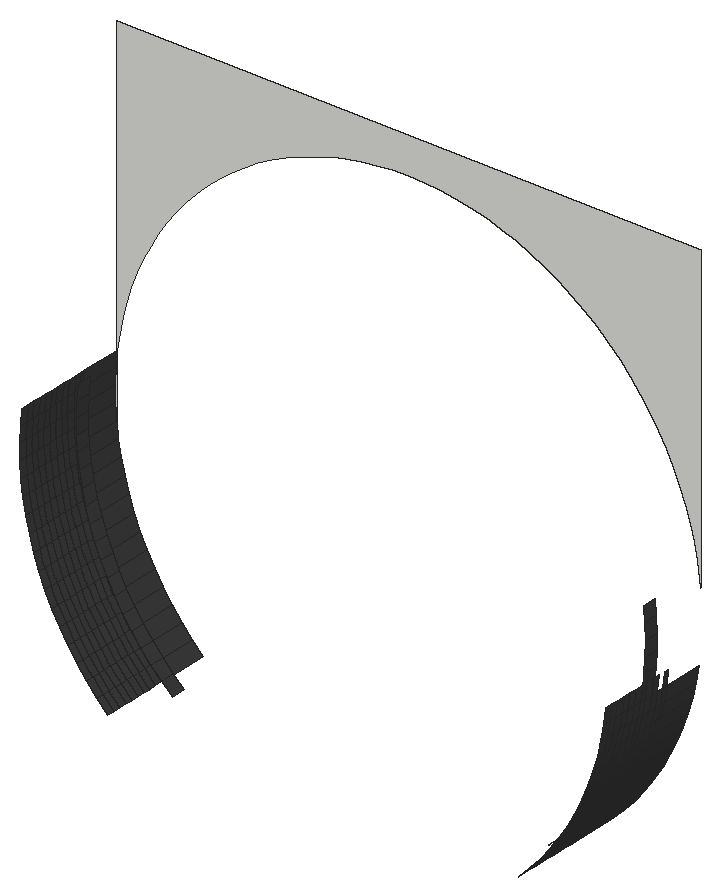
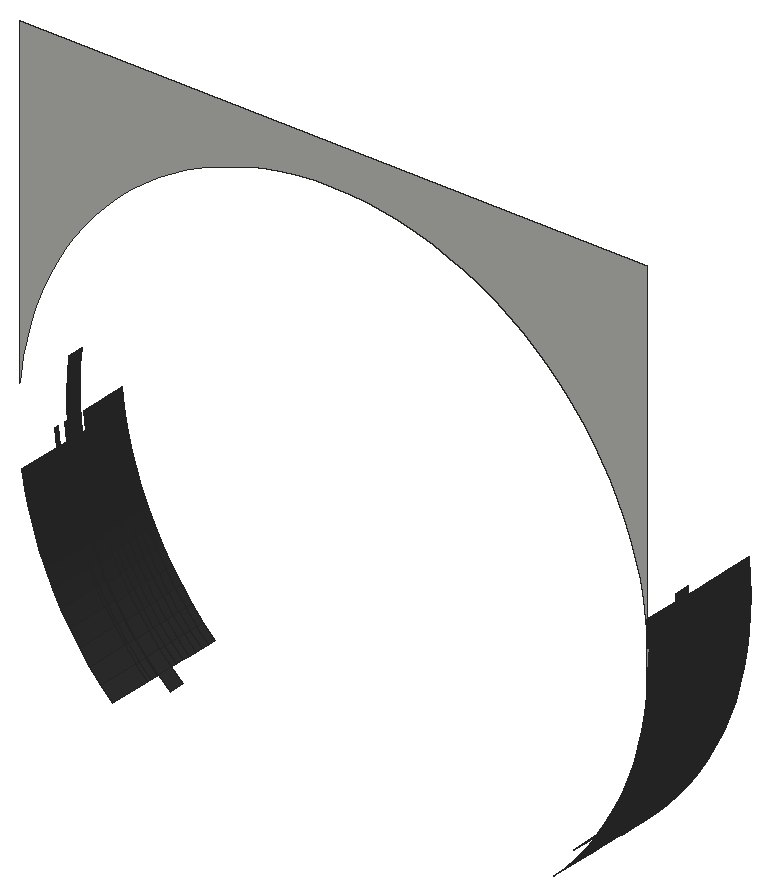
# SketchUp Ruby script. Lengths in inches.
U = 1.inch
M = Sketchup.active_model
def pt(a) = Geom::Point3d.new(a.map { |v| v * U })
def face(e, loops, mat)
  f = e.add_face(loops[0].map { |a| pt(a) })
  loops[1..].each { |l| e.add_face(l.map { |a| pt(a) }).erase! }
  f.material = f.back_material = mat if mat
  f
end
# faces: each face lists its corners as indices into pts; further lists are holes
def faces(e, pts, list, mat = nil) = list.each { |f| face(e, (f[0].is_a?(Array) ? f : [f]).map { |l| l.map { |i| pts[i] } }, mat) }
# xy, xz, yz: faces in a plane at the given z, y or x. An outline is a flat list of corners, or four numbers for a rectangle; further outlines are holes
def ring(l) = l.size == 4 ? [[l[0], l[1]], [l[2], l[1]], [l[2], l[3]], [l[0], l[3]]] : l.each_slice(2).to_a
def flat(e, list, mat, &to3) = list.each { |f| face(e, (f[0].is_a?(Array) ? f : [f]).map { |l| ring(l).map { |u, v| to3.(u, v) } }, mat) }
def xy(e, z, list, mat = nil) = flat(e, list, mat) { |x, y| [x, y, z] }
def xz(e, y, list, mat = nil) = flat(e, list, mat) { |x, z| [x, y, z] }
def yz(e, x, list, mat = nil) = flat(e, list, mat) { |y, z| [x, y, z] }
def lines(e, pts, list) = list.each { |a, b| e.add_line(pt(pts[a]), pt(pts[b])) }
# prism: a flat outline (further loops are holes) pulled along v
def prism(e, loops, v, mat = nil)
  f = face(e, loops, mat); d = Geom::Vector3d.new(v.map { |x| x * U })
  f.pushpull(f.normal.samedirection?(d) ? d.length : -d.length)
end
def box(e, o, s, mat = nil) = prism(e, [[o, [o[0] + s[0], o[1], o[2]], [o[0] + s[0], o[1] + s[1], o[2]], [o[0], o[1] + s[1], o[2]]]], [0, 0, s[2]], mat)
def at(x, y, z, deg = 0) = Geom::Transformation.translation(pt([x, y, z])) * Geom::Transformation.rotation(ORIGIN, Z_AXIS, deg.degrees)
def axes(o, x, y, z) = Geom::Transformation.new([*x, 0, *y, 0, *z, 0, *pt(o).to_a, 1])
def part(name) = M.definitions.add(name)
# library, detail: a bought-in or finely detailed component or shape, given as its bounding box
def library(name, o, s) = part(name).tap { |d| box(d.entities, o, s) }
def detail(e, o, s) = box(e.add_group.entities, o, s)
def put(e, d, t, mat = nil) = e.add_instance(d, t).tap { |i| i.material = mat if mat }
def group(e, t, mat = nil) = e.add_group.tap { |g| g.transformation = t; g.material = mat if mat }.entities
root = M.entities
M.materials.add("[Color M07]").color = [58, 58, 58]
xz(root,24,[[27.46,301.2,27.46,312.54,27.31,310.86,27.18,307.68,27.23,304.49,27.45,301.3125],[27.46,312.54,27.46,373.6875,145.46,373.6875,145.46,312.54,145.32,314.03,144.86,317.1875,144.22,320.31,143.42,323.39,142.46,326.43,141.33,329.41,140.05,332.33,138.61,335.17,137.02,337.93,135.28,340.6,133.4,343.17,131.39,345.64,129.25,348,126.98,350.24,124.6,352.36,122.1,354.34,119.51,356.1875,116.81,357.89,114.04,359.45,111.18,360.85,108.24,362.1,105.25,363.19,102.2,364.12,99.11,364.88,95.98,365.48,92.82,365.91,89.65,366.16,86.46,366.25,83.28,366.16,80.1,365.91,76.94,365.48,73.8125,364.88,70.72,364.12,67.67,363.19,64.68,362.1,61.75,360.85,58.89,359.45,56.11,357.89,53.42,356.1875,50.82,354.34,48.32,352.36,45.94,350.24,43.67,348,41.53,345.64,39.52,343.17,37.64,340.6,35.9,337.93,34.3125,335.17,32.875,332.33,31.59,329.41,30.46,326.43,29.5,323.39,28.7,320.31,28.06,317.1875,27.6,314.03]])
p = [[48.46,14.875,263.875],[46.2,14.875,265.98],[46.2,12,265.98],[48.46,12,263.875],[126.72,14.875,265.98],[124.46,14.875,263.875],
  [124.46,12,263.875],[126.72,12,265.98],[44.92,0,264.68],[44.92,1.5,264.68],[42.7,1.5,266.97],[42.7,0,266.97],
  [130.22,0,266.97],[130.22,1.5,266.97],[128.01,1.5,264.68],[128.01,0,264.68],[44.92,3,264.68],[42.7,3,266.97],
  [130.22,3,266.97],[128.01,3,264.68],[44.92,4.5,264.68],[42.7,4.5,266.97],[130.22,4.5,266.97],[128.01,4.5,264.68],
  [44.92,6,264.68],[42.7,6,266.97],[130.22,6,266.97],[128.01,6,264.68],[44.92,7.5,264.68],[42.7,7.5,266.97],
  [130.22,7.5,266.97],[128.01,7.5,264.68],[44.92,9,264.68],[42.7,9,266.97],[130.22,9,266.97],[128.01,9,264.68],
  [44.92,10.5,264.68],[42.7,10.5,266.97],[130.22,10.5,266.97],[128.01,10.5,264.68],[44.92,12,264.68],[42.7,12,266.97],
  [130.22,12,266.97],[128.01,12,264.68],[44.92,13.5,264.68],[42.7,13.5,266.97],[130.22,13.5,266.97],[128.01,13.5,264.68],
  [44.92,15,264.68],[42.7,15,266.97],[130.22,15,266.97],[128.01,15,264.68],[44.92,15.8125,264.68],[42.7,15.8125,266.97],
  [130.22,15.8125,266.97],[128.01,15.8125,264.68],[42.7,24,266.97],[44.92,24,264.68],[128.01,24,264.68],[130.22,24,266.97],
  [44.05,14.875,268.2],[44.05,12,268.2],[128.87,14.875,268.2],[128.87,12,268.2],[40.62,1.5,269.375],[40.62,0,269.375],
  [132.31,0,269.375],[132.31,1.5,269.375],[40.62,3,269.375],[132.31,3,269.375],[40.62,4.5,269.375],[132.31,4.5,269.375],
  [40.62,6,269.375],[132.31,6,269.375],[40.62,7.5,269.375],[132.31,7.5,269.375],[40.62,9,269.375],[132.31,9,269.375],
  [40.62,10.5,269.375],[132.31,10.5,269.375],[40.62,12,269.375],[132.31,12,269.375],[40.62,13.5,269.375],[132.31,13.5,269.375],
  [40.62,15,269.375],[132.31,15,269.375],[40.62,15.8125,269.375],[132.31,15.8125,269.375],[40.62,24,269.375],[132.31,24,269.375],
  [42.03,14.875,270.54],[42.03,12,270.54],[130.89,14.875,270.54],[130.89,12,270.54],[38.66,1.5,271.89],[38.66,0,271.89],
  [134.26,0,271.89],[134.26,1.5,271.89],[38.66,3,271.89],[134.26,3,271.89],[38.66,4.5,271.89],[134.26,4.5,271.89],
  [38.66,6,271.89],[134.26,6,271.89],[38.66,7.5,271.89],[134.26,7.5,271.89],[38.66,9,271.89],[134.26,9,271.89],
  [38.66,10.5,271.89],[134.26,10.5,271.89],[38.66,12,271.89],[134.26,12,271.89],[38.66,13.5,271.89],[134.26,13.5,271.89],
  [38.66,15,271.89],[134.26,15,271.89],[38.66,15.8125,271.89],[134.26,15.8125,271.89],[38.66,24,271.89],[134.26,24,271.89],
  [40.14,14.875,272.98],[40.14,12,272.98],[132.78,14.875,272.98],[132.78,12,272.98],[36.85,1.5,274.51],[36.85,0,274.51],
  [136.07,0,274.51],[136.07,1.5,274.51],[36.85,3,274.51],[136.07,3,274.51],[36.85,4.5,274.51],[136.07,4.5,274.51],
  [36.85,6,274.51],[136.07,6,274.51],[36.85,7.5,274.51],[136.07,7.5,274.51],[36.85,9,274.51],[136.07,9,274.51],
  [36.85,10.5,274.51],[136.07,10.5,274.51],[36.85,12,274.51],[136.07,12,274.51],[36.85,13.5,274.51],[136.07,13.5,274.51],
  [36.85,15,274.51],[136.07,15,274.51],[36.85,15.8125,274.51],[136.07,15.8125,274.51],[36.85,24,274.51],[136.07,24,274.51],
  [38.38,14.875,275.51],[38.38,12,275.51],[134.54,14.875,275.51],[134.54,12,275.51],[35.18,1.5,277.23],[35.18,0,277.23],
  [137.75,0,277.23],[137.75,1.5,277.23],[35.18,3,277.23],[137.75,3,277.23],[35.18,4.5,277.23],[137.75,4.5,277.23],
  [35.18,6,277.23],[137.75,6,277.23],[35.18,7.5,277.23],[137.75,7.5,277.23],[35.18,9,277.23],[137.75,9,277.23],
  [35.18,10.5,277.23],[137.75,10.5,277.23],[35.18,12,277.23],[137.75,12,277.23],[35.18,13.5,277.23],[137.75,13.5,277.23],
  [35.18,15,277.23],[137.75,15,277.23],[35.18,15.8125,277.23],[137.75,15.8125,277.23],[35.18,24,277.23],[137.75,24,277.23],
  [36.76,14.875,278.14],[36.76,12,278.14],[136.16,14.875,278.14],[136.16,12,278.14],[33.65,1.5,280.02],[33.65,0,280.02],
  [139.27,0,280.02],[139.27,1.5,280.02],[33.65,3,280.02],[139.27,3,280.02],[33.65,4.5,280.02],[139.27,4.5,280.02],
  [33.65,6,280.02],[139.27,6,280.02],[33.65,7.5,280.02],[139.27,7.5,280.02],[33.65,9,280.02],[139.27,9,280.02],
  [33.65,10.5,280.02],[139.27,10.5,280.02],[33.65,12,280.02],[139.27,12,280.02],[33.65,13.5,280.02],[139.27,13.5,280.02],
  [33.65,15,280.02],[139.27,15,280.02],[33.65,15.8125,280.02],[139.27,15.8125,280.02],[33.65,24,280.02],[139.27,24,280.02],
  [35.28,14.875,280.85],[35.28,12,280.85],[137.64,14.875,280.85],[137.64,12,280.85],[32.28,1.5,282.9],[32.28,0,282.9],
  [140.64,0,282.9],[140.64,1.5,282.9],[32.28,3,282.9],[140.64,3,282.9],[32.28,4.5,282.9],[140.64,4.5,282.9],
  [32.28,6,282.9],[140.64,6,282.9],[32.28,7.5,282.9],[140.64,7.5,282.9],[32.28,9,282.9],[140.64,9,282.9],
  [32.28,10.5,282.9],[140.64,10.5,282.9],[32.28,12,282.9],[140.64,12,282.9],[32.28,13.5,282.9],[140.64,13.5,282.9],
  [32.28,15,282.9],[140.64,15,282.9],[32.28,15.8125,282.9],[140.64,15.8125,282.9],[32.28,24,282.9],[140.64,24,282.9],
  [33.95,14.875,283.64],[33.95,12,283.64],[138.97,14.875,283.64],[138.97,12,283.64],[31.07,1.5,285.85],[31.07,0,285.85],
  [141.86,0,285.85],[141.86,1.5,285.85],[31.07,3,285.85],[141.86,3,285.85],[31.07,4.5,285.85],[141.86,4.5,285.85],
  [31.07,6,285.85],[141.86,6,285.85],[31.07,7.5,285.85],[141.86,7.5,285.85],[31.07,9,285.85],[141.86,9,285.85],
  [31.07,10.5,285.85],[141.86,10.5,285.85],[31.07,12,285.85],[141.86,12,285.85],[31.07,13.5,285.85],[141.86,13.5,285.85],
  [31.07,15,285.85],[141.86,15,285.85],[31.07,15.8125,285.85],[141.86,15.8125,285.85],[31.07,24,285.85],[141.86,24,285.85],
  [32.78,14.875,286.5],[32.78,12,286.5],[140.15,14.875,286.5],[140.15,12,286.5],[30.01,1.5,288.85],[30.01,0,288.85],
  [142.91,0,288.85],[142.91,1.5,288.85],[30.01,3,288.85],[142.91,3,288.85],[30.01,4.5,288.85],[142.91,4.5,288.85],
  [30.01,6,288.85],[142.91,6,288.85],[30.01,7.5,288.85],[142.91,7.5,288.85],[30.01,9,288.85],[142.91,9,288.85],
  [30.01,10.5,288.85],[142.91,10.5,288.85],[30.01,12,288.85],[142.91,12,288.85],[30.01,13.5,288.85],[142.91,13.5,288.85],
  [30.01,15,288.85],[142.91,15,288.85],[30.01,15.8125,288.85],[142.91,15.8125,288.85],[30.01,24,288.85],[142.91,24,288.85],
  [31.75,14.875,289.41],[31.75,12,289.41],[141.17,14.875,289.41],[141.17,12,289.41],[29.12,1.5,291.91],[29.12,0,291.91],
  [143.8,0,291.91],[143.8,1.5,291.91],[29.12,3,291.91],[143.8,3,291.91],[29.12,4.5,291.91],[143.8,4.5,291.91],
  [29.12,6,291.91],[143.8,6,291.91],[29.12,7.5,291.91],[143.8,7.5,291.91],[29.12,9,291.91],[143.8,9,291.91],
  [29.12,10.5,291.91],[143.8,10.5,291.91],[29.12,12,291.91],[143.8,12,291.91],[29.12,13.5,291.91],[143.8,13.5,291.91],
  [29.12,15,291.91],[143.8,15,291.91],[29.12,15.8125,291.91],[143.8,15.8125,291.91],[29.12,24,291.91],[143.8,24,291.91],
  [30.89,14.875,292.375],[30.89,12,292.375],[142.03,14.875,292.375],[142.03,12,292.375],[28.39,1.5,295.01],[28.39,0,295.01],
  [144.53,0,295.01],[144.53,1.5,295.01],[28.39,3,295.01],[144.53,3,295.01],[28.39,4.5,295.01],[144.53,4.5,295.01],
  [28.39,6,295.01],[144.53,6,295.01],[28.39,7.5,295.01],[144.53,7.5,295.01],[28.39,9,295.01],[144.53,9,295.01],
  [28.39,10.5,295.01],[144.53,10.5,295.01],[28.39,12,295.01],[144.53,12,295.01],[28.39,13.5,295.01],[144.53,13.5,295.01],
  [28.39,15,295.01],[144.53,15,295.01],[28.39,15.8125,295.01],[144.53,15.8125,295.01],[28.39,24,295.01],[144.53,24,295.01],
  [30.1875,14.875,295.38],[30.1875,12,295.38],[142.74,14.875,295.38],[142.74,12,295.38],[27.84,1.5,298.15],[27.84,0,298.15],
  [145.09,0,298.15],[145.09,1.5,298.15],[27.84,3,298.15],[145.09,3,298.15],[27.84,4.5,298.15],[145.09,4.5,298.15],
  [27.84,6,298.15],[145.09,6,298.15],[27.84,7.5,298.15],[145.09,7.5,298.15],[27.84,9,298.15],[145.09,9,298.15],
  [27.84,10.5,298.15],[145.09,10.5,298.15],[27.84,12,298.15],[145.09,12,298.15],[27.84,13.5,298.15],[145.09,13.5,298.15],
  [27.84,15,298.15],[145.09,15,298.15],[27.84,15.8125,298.15],[145.09,15.8125,298.15],[27.84,24,298.15],[145.09,24,298.15],
  [29.65,14.875,298.42],[29.65,12,298.42],[143.28,14.875,298.42],[143.28,12,298.42],[27.45,1.5,301.3125],[27.45,0,301.3125],
  [145.47,0,301.3125],[145.47,1.5,301.3125],[27.45,3,301.3125],[145.47,3,301.3125],[27.45,4.5,301.3125],[145.47,4.5,301.3125],
  [27.45,6,301.3125],[145.47,6,301.3125],[27.45,7.5,301.3125],[145.47,7.5,301.3125],[27.45,9,301.3125],[145.47,9,301.3125],
  [27.45,10.5,301.3125],[27.45,12,301.3125],[145.47,10.5,301.3125],[145.47,12,301.3125],[27.45,13.5,301.3125],[145.47,13.5,301.3125],
  [27.45,15,301.3125],[27.45,15.8125,301.3125],[145.47,15.8125,301.3125],[145.47,15,301.3125],[27.45,24,301.3125],[27.46,24,301.2],
  [29.27,14.875,301.49],[29.27,12,301.49],[143.65,14.875,301.49],[143.65,12,301.49],[27.23,1.5,304.49],[27.23,0,304.49],
  [27.23,3,304.49],[27.23,4.5,304.49],[27.23,6,304.49],[27.23,7.5,304.49],[27.23,9,304.49],[27.23,10.5,304.49],
  [27.23,12,304.49],[27.23,13.5,304.49],[27.23,15,304.49],[27.23,15.8125,304.49],[27.23,24,304.49],[29.06,14.875,304.57],
  [29.06,12,304.57],[143.87,14.875,304.57],[143.87,12,304.57],[27.18,1.5,307.68],[27.18,0,307.68],[27.18,3,307.68],
  [27.18,4.5,307.68],[27.18,6,307.68],[27.18,7.5,307.68],[27.18,9,307.68],[27.18,10.5,307.68],[27.18,12,307.68],
  [27.18,13.5,307.68],[27.18,15,307.68],[27.18,15.8125,307.68],[27.18,24,307.68],[29.01,14.875,307.66],[29.01,12,307.66],
  [143.91,14.875,307.66],[143.91,12,307.66],[27.31,1.5,310.86],[27.31,0,310.86],[27.31,3,310.86],[27.31,4.5,310.86],
  [27.31,6,310.86],[27.31,7.5,310.86],[27.31,9,310.86],[27.31,10.5,310.86],[27.31,12,310.86],[27.31,13.5,310.86],
  [29.13,14.875,310.74],[29.13,12,310.74],[143.79,14.875,310.74],[143.79,12,310.74],[27.31,15,310.86],[27.31,15.8125,310.86],
  [27.31,24,310.86],[29.42,14.875,313.82],[29.42,12,313.82],[143.51,14.875,313.82],[143.51,12,313.82],[27.6,1.5,314.03],
  [27.6,0,314.03],[27.6,3,314.03],[27.6,4.5,314.03],[27.6,6,314.03],[27.6,7.5,314.03],[27.6,9,314.03],
  [27.6,10.5,314.03],[27.6,12,314.03],[27.6,13.5,314.03],[27.6,15,314.03],[27.6,15.8125,314.03],[27.6,24,314.03],
  [27.46,24,312.54]]
faces(root,p,[[0,1,2,3],[4,5,6,7],[8,9,10,11],[12,13,14,15],[9,16,17,10],[13,18,19,14],[16,20,21,17],[18,22,23,19],
  [20,24,25,21],[22,26,27,23],[24,28,29,25],[26,30,31,27],[28,32,33,29],[30,34,35,31],[32,36,37,33],[34,38,39,35],
  [36,40,41,37],[38,42,43,39],[44,40,41,45],[46,42,43,47],[48,44,45,49],[50,46,47,51],[52,53,49,48],[54,55,51,50],
  [56,53,52,57],[58,55,54,59],[1,60,61,2],[62,4,7,63],[11,10,64,65],[66,67,13,12],[10,17,68,64],[67,69,18,13],
  [17,21,70,68],[69,71,22,18],[21,25,72,70],[71,73,26,22],[25,29,74,72],[73,75,30,26],[29,33,76,74],[75,77,34,30],
  [33,37,78,76],[77,79,38,34],[37,41,80,78],[79,81,42,38],[45,41,80,82],[83,81,42,46],[49,45,82,84],[85,83,46,50],
  [53,86,84,49],[87,54,50,85],[88,86,53,56],[59,54,87,89],[60,90,91,61],[92,62,63,93],[65,64,94,95],[96,97,67,66],
  [64,68,98,94],[97,99,69,67],[68,70,100,98],[99,101,71,69],[70,72,102,100],[101,103,73,71],[72,74,104,102],[103,105,75,73],
  [74,76,106,104],[105,107,77,75],[76,78,108,106],[107,109,79,77],[78,80,110,108],[109,111,81,79],[82,80,110,112],[113,111,81,83],
  [84,82,112,114],[115,113,83,85],[86,116,114,84],[117,87,85,115],[118,116,86,88],[89,87,117,119],[90,120,121,91],[122,92,93,123],
  [95,94,124,125],[126,127,97,96],[94,98,128,124],[127,129,99,97],[98,100,130,128],[129,131,101,99],[100,102,132,130],[131,133,103,101],
  [102,104,134,132],[133,135,105,103],[104,106,136,134],[135,137,107,105],[106,108,138,136],[137,139,109,107],[108,110,140,138],[139,141,111,109],
  [112,110,140,142],[143,141,111,113],[114,112,142,144],[145,143,113,115],[116,146,144,114],[147,117,115,145],[148,146,116,118],[119,117,147,149],
  [120,150,151,121],[152,122,123,153],[125,124,154,155],[156,157,127,126],[124,128,158,154],[157,159,129,127],[128,130,160,158],[159,161,131,129],
  [130,132,162,160],[161,163,133,131],[132,134,164,162],[163,165,135,133],[134,136,166,164],[165,167,137,135],[136,138,168,166],[167,169,139,137],
  [138,140,170,168],[169,171,141,139],[142,140,170,172],[173,171,141,143],[144,142,172,174],[175,173,143,145],[146,176,174,144],[177,147,145,175],
  [178,176,146,148],[149,147,177,179],[150,180,181,151],[182,152,153,183],[155,154,184,185],[186,187,157,156],[154,158,188,184],[187,189,159,157],
  [158,160,190,188],[189,191,161,159],[160,162,192,190],[191,193,163,161],[162,164,194,192],[193,195,165,163],[164,166,196,194],[195,197,167,165],
  [166,168,198,196],[197,199,169,167],[168,170,200,198],[199,201,171,169],[172,170,200,202],[203,201,171,173],[174,172,202,204],[205,203,173,175],
  [176,206,204,174],[207,177,175,205],[208,206,176,178],[179,177,207,209],[180,210,211,181],[212,182,183,213],[185,184,214,215],[216,217,187,186],
  [184,188,218,214],[217,219,189,187],[188,190,220,218],[219,221,191,189],[190,192,222,220],[221,223,193,191],[192,194,224,222],[223,225,195,193],
  [194,196,226,224],[225,227,197,195],[196,198,228,226],[227,229,199,197],[198,200,230,228],[229,231,201,199],[202,200,230,232],[233,231,201,203],
  [204,202,232,234],[235,233,203,205],[206,236,234,204],[237,207,205,235],[238,236,206,208],[209,207,237,239],[210,240,241,211],[242,212,213,243],
  [215,214,244,245],[246,247,217,216],[214,218,248,244],[247,249,219,217],[218,220,250,248],[249,251,221,219],[220,222,252,250],[251,253,223,221],
  [222,224,254,252],[253,255,225,223],[224,226,256,254],[255,257,227,225],[226,228,258,256],[257,259,229,227],[228,230,260,258],[259,261,231,229],
  [232,230,260,262],[263,261,231,233],[234,232,262,264],[265,263,233,235],[236,266,264,234],[267,237,235,265],[268,266,236,238],[239,237,267,269],
  [240,270,271,241],[272,242,243,273],[245,244,274,275],[276,277,247,246],[244,248,278,274],[277,279,249,247],[248,250,280,278],[279,281,251,249],
  [250,252,282,280],[281,283,253,251],[252,254,284,282],[283,285,255,253],[254,256,286,284],[285,287,257,255],[256,258,288,286],[287,289,259,257],
  [258,260,290,288],[289,291,261,259],[262,260,290,292],[293,291,261,263],[264,262,292,294],[295,293,263,265],[266,296,294,264],[297,267,265,295],
  [298,296,266,268],[269,267,297,299],[270,300,301,271],[302,272,273,303],[275,274,304,305],[306,307,277,276],[274,278,308,304],[307,309,279,277],
  [278,280,310,308],[309,311,281,279],[280,282,312,310],[311,313,283,281],[282,284,314,312],[313,315,285,283],[284,286,316,314],[315,317,287,285],
  [286,288,318,316],[317,319,289,287],[288,290,320,318],[319,321,291,289],[292,290,320,322],[323,321,291,293],[294,292,322,324],[325,323,293,295],
  [296,326,324,294],[327,297,295,325],[328,326,296,298],[299,297,327,329],[300,330,331,301],[332,302,303,333],[305,304,334,335],[336,337,307,306],
  [304,308,338,334],[337,339,309,307],[308,310,340,338],[339,341,311,309],[310,312,342,340],[341,343,313,311],[312,314,344,342],[343,345,315,313],
  [314,316,346,344],[345,347,317,315],[316,318,348,346],[347,349,319,317],[318,320,350,348],[349,351,321,319],[322,320,350,352],[353,351,321,323],
  [324,322,352,354],[355,353,323,325],[326,356,354,324],[357,327,325,355],[358,356,326,328],[329,327,357,359],[330,360,361,331],[362,332,333,363],
  [335,334,364,365],[366,367,337,336],[334,338,368,364],[367,369,339,337],[338,340,370,368],[369,371,341,339],[340,342,372,370],[371,373,343,341],
  [342,344,374,372],[373,375,345,343],[344,346,376,374],[375,377,347,345],[346,348,378,376],[377,379,349,347],[348,350,380,378],[379,381,351,349],
  [352,350,380,382],[383,381,351,353],[354,352,382,384],[385,383,353,355],[356,386,384,354],[387,357,355,385],[388,386,356,358],[359,357,387,389],
  [360,390,391,361],[392,362,363,393],[365,364,394,395],[396,397,367,366],[364,368,398,394],[397,399,369,367],[368,370,400,398],[399,401,371,369],
  [370,372,402,400],[401,403,373,371],[372,374,404,402],[403,405,375,373],[374,376,406,404],[405,407,377,375],[376,378,408,406],[378,380,409,408],
  [410,411,381,379],[382,380,409,412],[413,411,381,383],[384,382,412,414],[386,415,414,384],[416,387,385,417],[418,415,386,388,419],[390,420,421,391],
  [422,392,393,423],[395,394,424,425],[394,398,426,424],[398,400,427,426],[400,402,428,427],[402,404,429,428],[404,406,430,429],[406,408,431,430],
  [408,409,432,431],[412,409,432,433],[414,412,433,434],[415,435,434,414],[436,435,415,418],[420,437,438,421],[439,422,423,440],[425,424,441,442],
  [424,426,443,441],[426,427,444,443],[427,428,445,444],[428,429,446,445],[429,430,447,446],[430,431,448,447],[431,432,449,448],[433,432,449,450],
  [434,433,450,451],[435,452,451,434],[453,452,435,436],[437,454,455,438],[456,439,440,457],[442,441,458,459],[441,443,460,458],[443,444,461,460],
  [444,445,462,461],[445,446,463,462],[446,447,464,463],[447,448,465,464],[448,449,466,465],[450,449,466,467],[454,468,469,455],[470,456,457,471],
  [451,450,467,472],[452,473,472,451],[474,473,452,453],[468,475,476,469],[477,470,471,478],[459,458,479,480],[458,460,481,479],[460,461,482,481],
  [461,462,483,482],[462,463,484,483],[463,464,485,484],[464,465,486,485],[465,466,487,486],[467,466,487,488],[472,467,488,489],[473,490,489,472],
  [491,490,473,474,492]],"[Color M07]")
